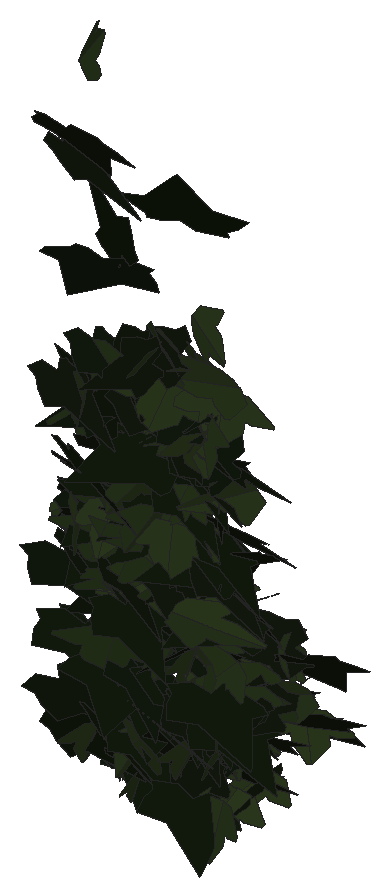
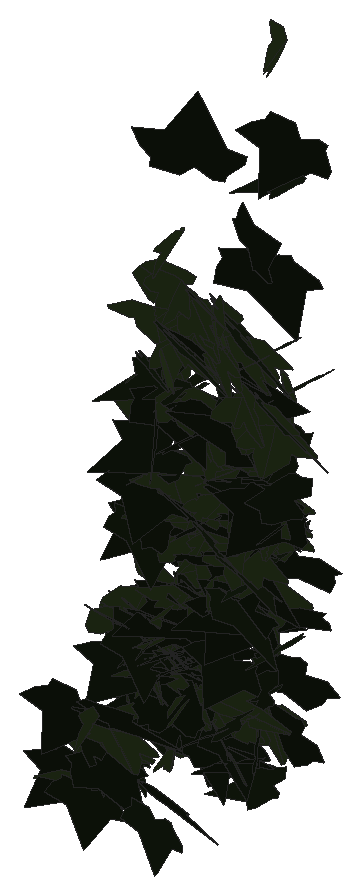
# SketchUp Ruby script. Lengths in millimetres.
U = 1.mm
M = Sketchup.active_model
def pt(a) = Geom::Point3d.new(a.map { |v| v * U })
def face(e, loops, mat)
  f = e.add_face(loops[0].map { |a| pt(a) })
  loops[1..].each { |l| e.add_face(l.map { |a| pt(a) }).erase! }
  f.material = f.back_material = mat if mat
  f
end
# faces: each face lists its corners as indices into pts; further lists are holes
def faces(e, pts, list, mat = nil) = list.each { |f| face(e, (f[0].is_a?(Array) ? f : [f]).map { |l| l.map { |i| pts[i] } }, mat) }
# xy, xz, yz: faces in a plane at the given z, y or x. An outline is a flat list of corners, or four numbers for a rectangle; further outlines are holes
def ring(l) = l.size == 4 ? [[l[0], l[1]], [l[2], l[1]], [l[2], l[3]], [l[0], l[3]]] : l.each_slice(2).to_a
def flat(e, list, mat, &to3) = list.each { |f| face(e, (f[0].is_a?(Array) ? f : [f]).map { |l| ring(l).map { |u, v| to3.(u, v) } }, mat) }
def xy(e, z, list, mat = nil) = flat(e, list, mat) { |x, y| [x, y, z] }
def xz(e, y, list, mat = nil) = flat(e, list, mat) { |x, z| [x, y, z] }
def yz(e, x, list, mat = nil) = flat(e, list, mat) { |y, z| [x, y, z] }
def lines(e, pts, list) = list.each { |a, b| e.add_line(pt(pts[a]), pt(pts[b])) }
# prism: a flat outline (further loops are holes) pulled along v
def prism(e, loops, v, mat = nil)
  f = face(e, loops, mat); d = Geom::Vector3d.new(v.map { |x| x * U })
  f.pushpull(f.normal.samedirection?(d) ? d.length : -d.length)
end
def box(e, o, s, mat = nil) = prism(e, [[o, [o[0] + s[0], o[1], o[2]], [o[0] + s[0], o[1] + s[1], o[2]], [o[0], o[1] + s[1], o[2]]]], [0, 0, s[2]], mat)
def at(x, y, z, deg = 0) = Geom::Transformation.translation(pt([x, y, z])) * Geom::Transformation.rotation(ORIGIN, Z_AXIS, deg.degrees)
def axes(o, x, y, z) = Geom::Transformation.new([*x, 0, *y, 0, *z, 0, *pt(o).to_a, 1])
def part(name) = M.definitions.add(name)
# library, detail: a bought-in or finely detailed component or shape, given as its bounding box
def library(name, o, s) = part(name).tap { |d| box(d.entities, o, s) }
def detail(e, o, s) = box(e.add_group.entities, o, s)
def put(e, d, t, mat = nil) = e.add_instance(d, t).tap { |i| i.material = mat if mat }
def group(e, t, mat = nil) = e.add_group.tap { |g| g.transformation = t; g.material = mat if mat }.entities
root = M.entities
M.materials.add("efeu1").color = [18, 25, 13]
M.materials.add("efeu2").color = [43, 57, 29]
c1 = part("ivyleaf_9")
p = [[39.1,54.8,31.7],[34.5,51.8,30.2],[-5.3,25.2,17.3],[-17.9,28.3,20.9],[-21.6,21.7,17],[-20.2,4.3,5.3],
  [-22.9,-0.3,2.5],[-17.1,-4,-0.6],[-2,-2.1,-1.2],[-0.7,-15.4,-10.1],[16.6,-22.3,-16.7],[21.1,-15.1,-12.5],
  [32.7,-10.7,-11],[46.1,-1.8,-6.6],[30.8,11.2,3.8]]
faces(c1.entities,p,[[0,1,2,3,4,5,6,7,8,9,10,11,12,13,14]],"efeu1")
c2 = part("ivyleaf_10")
p = [[0,12.8,-0.8],[-1.5,51.3,-10.9],[-4.9,51,-11.6],[-13.6,26.5,-7.3],[-13.2,15.9,-4.6],[-21.1,19.3,-7.2],
  [-29.5,16.3,-8.3],[-29.2,8.3,-6.2],[-19.7,-9.8,0.5],[-7.6,-13,4],[1,-12.2,5.8],[-0.4,51.1,-11.1],
  [-1.5,51.1,-10.9],[1,-12.4,5.9],[16.9,-12.4,3.5],[35.1,9.1,-5.1],[35,12.9,-6.1],[20.5,16.4,-4.9],
  [15.8,15,-3.8],[15.3,27.6,-7.1],[12.8,31.3,-7.8]]
faces(c2.entities,p,[[0,1,2,3,4,5,6,7,8,9,10],[11,12,0,13,14,15,16,17,18,19,20]],"efeu2")
put(root,c1,axes([3061,972.3,1635.7],[1.11104,-0.60833,-0.00442],[0.18227,0.09795,-0.83193],[1.14337,0.57552,0.13692]))
put(root,c1,axes([3073,929.3,1931.4],[0.51198,-0.71925,-0.46522],[-0.31436,0.43492,-0.7679],[1.59967,0.31566,-0.00201]))
put(root,c2,axes([3095.9,929.4,1935.7],[-1.34679,0.48513,0.2721],[-0.40759,0.16873,-0.8578],[-0.97701,-0.73914,-0.01723]))
put(root,c1,axes([3071.8,944.6,1785],[0.22855,-0.87259,0.06119],[0.01219,-0.06088,-0.88081],[1.66474,0.12024,-0.00195]))
put(root,c2,axes([3094.9,925.5,1684.9],[-0.36174,-0.88496,-0.00511],[0.00062,0.00516,-0.90514],[1.68428,-0.19007,-0.00076]))
put(root,c1,axes([3112.5,915.7,2059.2],[-1.31576,0.6085,-0.06336],[0.07292,-0.05235,-0.92089],[-1.16208,-0.69226,0.01395]))
put(root,c2,axes([3090.5,929.2,2034.6],[-1.18294,-0.64557,-0.1632],[0.34038,0.05319,-0.89158],[1.22074,-0.64042,0.09046]))
put(root,c1,axes([3058.2,928.1,1680.8],[0.22802,-0.13014,-0.86664],[1.59305,0.27606,0.07426],[0.49399,-0.83019,0.16055]))
put(root,c1,axes([3074.9,894.8,2090.1],[0.54567,-0.85198,-0.28202],[0.00984,0.29762,-0.89387],[1.70799,0.27047,0.09525]))
put(root,c2,axes([3088.3,929.8,1926.4],[1.70167,-0.0799,0.05219],[0.0972,-0.01482,-0.89762],[0.15343,0.89551,-0.01019]))
put(root,c1,axes([3084.1,933.4,1947.3],[1.61846,0.33248,-0.06095],[-0.10872,-0.02127,-0.91307],[-0.63407,0.8523,0.00099]))
put(root,c1,axes([3120.6,1097.6,1663.8],[-1.47036,0.30855,0.01572],[-0.04089,-0.01141,-0.8317],[-0.58657,-0.77265,0.01856]))
put(root,c2,axes([3102.9,891.1,2078.3],[0.7245,-0.79091,-0.40343],[-0.06508,0.42556,-0.86657],[1.68853,0.35576,0.1397]))
put(root,c2,axes([3100.7,886.1,1936.8],[0.35936,-0.41507,-0.79085],[0.11802,0.81247,-0.41162],[1.69576,0.03142,0.19624]))
put(root,c2,axes([3102.9,929.8,1928.9],[-1.33956,-0.59327,0.01785],[0.22886,-0.16965,-0.8969],[1.10619,-0.68333,0.20718]))
put(root,c1,axes([3093.5,884.1,2377.9],[1.73709,0.16773,-0.33496],[-0.65268,0.0191,-0.92489],[-0.28691,0.97206,0.07597]))
put(root,c1,axes([3079.3,905.2,1882],[-0.56523,-0.36346,-0.83752],[1.15093,0.5815,-0.46679],[1.30176,-0.67194,0.04905]))
put(root,c2,axes([3104.4,933.3,1801.8],[0.54825,0.78096,-0.33312],[-0.46526,-0.26058,-0.82231],[-1.54746,0.35503,0.12921]))
put(root,c1,axes([3110.6,1107.5,1633.5],[0.18597,0.77027,0.27647],[0.04997,0.27534,-0.7764],[-1.55675,0.10086,0.00811]))
put(root,c1,axes([3072.7,904,1738.3],[0.14565,-0.1347,-0.92948],[1.05057,0.76094,-0.06482],[1.44614,-0.53922,0.14071]))
put(root,c1,axes([3067.2,929.1,1966.6],[1.22331,-0.50011,0.43505],[0.86633,-0.10748,-0.79609],[0.91703,0.76867,0.17173]))
put(root,c1,axes([3082.7,906.4,1900.5],[1.00727,-0.69391,-0.2124],[-0.12161,0.2173,-0.86916],[1.37577,0.52725,0.07868]))
put(root,c1,axes([3086.3,963.9,1668.5],[0.14607,-0.13064,-0.83273],[1.33119,-0.45676,0.13612],[-0.89526,-0.7005,0.06654]))
put(root,c1,axes([3123.1,952,1829.2],[-0.2636,0.86615,-0.01475],[-0.29797,-0.03972,-0.86228],[-1.62155,-0.1335,0.16085]))
put(root,c1,axes([3117,908.7,2227.7],[0.90471,0.57918,-0.65463],[-0.8303,-0.48851,-0.749],[-1.4415,0.64489,0.02056]))
put(root,c1,axes([3080.1,899.8,2348.9],[1.09753,-0.76119,-0.19476],[0.03349,0.25404,-0.94077],[1.49499,0.55313,0.16406]))
put(root,c2,axes([3130.3,933.5,2066.3],[-0.60089,0.22129,0.83082],[-1.31041,0.465,-0.3855],[-0.98001,-0.75744,0.00606]))
put(root,c2,axes([3111.9,971.8,1651.5],[0.73007,-0.73576,0.02906],[0.02388,-0.02624,-0.82975],[1.40119,0.3838,-0.001]))
put(root,c1,axes([3138.8,901.2,2059.6],[-0.123,0.12449,0.9838],[-0.86939,0.87132,-0.14026],[-1.67514,-0.46135,0.00056]))
put(root,c1,axes([3120.6,959.4,1669.9],[0.19457,0.83622,-0.0593],[-0.01111,-0.05903,-0.84245],[-1.59546,0.10239,-0.00137]))
put(root,c1,axes([3098.2,905.3,1808.6],[-0.69692,-0.70373,-0.51272],[0.58025,0.41737,-0.79061],[1.55221,-0.47199,0.06534]))
put(root,c2,axes([3145,958.9,1708.5],[0.5784,0.03428,-0.94877],[-1.80391,0.06804,-0.30115],[0.10354,0.99393,0.05334]))
put(root,c1,axes([3133.9,923.6,1853.6],[0.04767,0.69432,0.56069],[-0.62264,0.52901,-0.64047],[-1.58025,-0.18749,0.26927]))
put(root,c1,axes([3098.5,928.2,1902],[0.13666,-0.89474,-0.00496],[-0.01012,0.00455,-0.8976],[1.70286,0.07183,-0.00494]))
put(root,c1,axes([3086.9,901.3,2000.8],[1.00367,-0.78971,0.23886],[0.19765,-0.21769,-0.94901],[1.55773,0.53644,-0.03348]))
put(root,c1,axes([3135.7,912.6,2244.2],[0.09116,-0.18226,1.01157],[-0.33332,0.99641,0.18782],[-1.92762,-0.18092,0.01536]))
put(root,c2,axes([3121.8,927.8,2054.8],[-1.52392,-0.43922,-0.06667],[0.10154,0.04135,-0.91321],[0.83938,-0.80242,-0.01057]))
put(root,c2,axes([3123.6,939.6,1880.2],[-1.65964,-0.15999,0.0083],[-0.00698,-0.02598,-0.88623],[0.30482,-0.87168,0.02489]))
put(root,c2,axes([3128.5,872.9,2477.3],[0.02596,-0.0121,1.00923],[-0.79646,0.9184,0.01667],[-1.748,-0.41864,0.00739]))
put(root,c1,axes([3110.7,953.2,1818.5],[1.31686,0.53596,0.01849],[0.00591,0.02618,-0.87502],[-1.02064,0.69167,0.01879]))
put(root,c2,axes([3129.7,895.4,1934.1],[-1.50138,-0.39575,0.18638],[-0.24418,-0.15811,-0.87876],[0.79592,-0.79502,0.08199]))
put(root,c1,axes([3111.1,907.3,1939.5],[1.41938,0.6399,0.01935],[0.02818,0.01246,-0.98269],[-1.21809,0.74594,-0.00019]))
put(root,c2,axes([3137,911.3,2119.3],[-1.607,0.10526,0.34407],[-0.67932,-0.13427,-0.83486],[-0.08643,-0.90184,0.16446]))
put(root,c1,axes([3097.2,935.3,1721.3],[1.12373,-0.62037,0.05149],[0.06616,-0.03799,-0.85643],[1.18289,0.59146,-0.00101]))
put(root,c1,axes([3132.4,918.3,1914.4],[-1.46169,-0.46735,0.06719],[-0.10838,-0.03568,-0.89903],[0.89204,-0.77013,0.00088]))
put(root,c1,axes([3110.7,976.4,1645.8],[-0.21903,-0.77726,-0.26],[0.12631,0.25285,-0.78526],[1.55472,-0.13004,0.02717]))
put(root,c1,axes([3103.7,914.4,2127.5],[0.51371,-0.87248,-0.2569],[-0.03673,0.26242,-0.9115],[1.73059,0.26455,0.05691]))
put(root,c1,axes([3138.6,919.1,1954.7],[-1.51094,-0.41525,0.13081],[-0.1992,-0.08203,-0.89562],[0.80429,-0.80041,0.02392]))
put(root,c2,axes([3117.8,958.1,1682.4],[1.32683,0.4648,0.13844],[0.06979,0.19121,-0.82664],[-0.92037,0.68457,0.1369]))
put(root,c2,axes([3132.1,923,1812.9],[-0.05377,-0.92668,0.01137],[0.00048,-0.01139,-0.92711],[1.76378,-0.02825,0.0006]))
put(root,c1,axes([3151.5,912.4,2131.1],[-1.07847,0.72273,0.07352],[-0.06021,0.06861,-0.91823],[-1.38129,-0.56728,-0.01738]))
put(root,c1,axes([3106.1,948.3,1824.4],[1.48155,0.22839,0.34224],[0.5744,0.18081,-0.80715],[-0.53221,0.83092,0.08157]))
put(root,c2,axes([3144.9,908.3,1951.1],[-1.56219,-0.25882,0.28159],[-0.52538,-0.06056,-0.86033],[0.50383,-0.86566,-0.024]))
put(root,c1,axes([3154,929.2,1857.8],[0.35816,0.19068,-0.91303],[-1.15512,-0.68222,-0.26758],[-1.34793,0.6353,-0.0133]))
put(root,c1,axes([3129.7,950.7,1755.1],[0.74558,0.7292,0.29822],[0.22493,0.27489,-0.82741],[-1.48242,0.40846,0.02444]))
put(root,c2,axes([3130.1,905.8,1949.7],[0.97186,0.72235,-0.26572],[-0.29912,-0.2143,-0.88461],[-1.43398,0.53427,0.00443]))
put(root,c2,axes([3123.6,929.1,1802.8],[0.12648,-0.47004,-0.76344],[0.16192,-0.75877,0.47458],[-1.69859,-0.10733,-0.01161]))
put(root,c2,axes([3144,892.5,1813.9],[-1.61379,-0.54917,0.14085],[-0.21586,-0.08397,-1.0102],[1.05719,-0.85544,0.00874]))
put(root,c1,axes([3111.5,964.5,1696.6],[0.82638,-0.73922,0.02209],[0.086,0.00095,-0.85641],[1.40489,0.43477,0.03943]))
put(root,c1,axes([3111.7,915.8,1704.7],[0.81271,-0.75705,0.14353],[0.16581,-0.11561,-0.86897],[1.45708,0.43541,0.01883]))
put(root,c1,axes([3132.8,967.3,1654.2],[-1.21543,-0.48621,-0.27967],[0.57464,0.05916,-0.79233],[0.89966,-0.69466,0.12827]))
put(root,c2,axes([3135.7,967.1,1675.2],[0.73068,-0.73868,0.14378],[0.16213,-0.11771,-0.83223],[1.42303,0.3927,0.02099]))
put(root,c1,axes([3117.1,944.3,1852.5],[0.64897,-0.82183,-0.03042],[0.09772,0.05414,-0.88715],[1.56212,0.33803,0.06813]))
put(root,c1,axes([3155.2,897.7,2031.3],[-0.07601,0.92139,0.12156],[0.03019,0.12233,-0.92202],[-1.76852,-0.03751,-0.02097]))
put(root,c2,axes([3151.2,931.1,1898.5],[1.5485,-0.00082,-0.37135],[-0.66747,0.29233,-0.76905],[0.23235,0.84524,0.26562]))
put(root,c1,axes([3153.8,962.4,1654.5],[0.07686,0.83589,-0.07013],[0.02354,-0.0708,-0.83671],[-1.59627,0.0392,-0.01572]))
put(root,c2,axes([3147.1,928.3,1652],[0.21499,-0.82793,-0.16248],[0.04035,0.16666,-0.8345],[1.60526,0.10669,0.04274]))
put(root,c1,axes([3157.4,936.6,1897.5],[-1.66892,-0.14765,-0.1341],[0.24926,0.02979,-0.88921],[0.2863,-0.8866,-0.00754]))
put(root,c2,axes([3139.7,899.1,1886.2],[-1.09838,-0.58599,-0.40281],[0.62694,0.23944,-0.82029],[1.19937,-0.66182,0.05989]))
put(root,c1,axes([3144.8,903.3,1775.8],[-0.97084,-0.73714,-0.09526],[0.07333,0.08916,-0.89623],[1.41269,-0.51121,-0.01895]))
put(root,c1,axes([3134.7,972.8,1673.8],[-0.11032,-0.84044,-0.02442],[0.02876,0.02343,-0.84233],[1.59994,-0.05837,0.01346]))
put(root,c2,axes([3151.1,941.6,1833],[-0.35364,-0.86964,0.05641],[0.04459,-0.06264,-0.88855],[1.65798,-0.18381,0.03593]))
put(root,c2,axes([3168.5,900.7,1705.4],[-1.21905,0.30898,0.61131],[-1.0852,0.22322,-0.71027],[-0.72232,-0.85682,0.03541]))
put(root,c1,axes([3114.8,916.2,2008.2],[0.69178,-0.13118,0.84205],[1.62042,0.09526,-0.35269],[-0.06974,0.91219,0.15792]))
put(root,c2,axes([3167.2,967.6,1694.2],[-0.11911,0.06884,-0.8475],[-0.65793,0.77433,0.08843],[1.4785,0.35012,-0.02893]))
put(root,c2,axes([3188,971.6,1665.5],[-0.73938,-0.14463,0.9129],[-1.64359,-0.29611,-0.41442],[0.62691,-0.9469,-0.00984]))
put(root,c2,axes([3164.9,909.8,1998.4],[-0.63705,-0.75707,0.42071],[-0.25793,-0.39969,-0.82709],[1.62808,-0.35956,0.03358]))
put(root,c2,axes([3158.1,917.5,1699.9],[-0.34064,-0.74572,0.42865],[0.08247,-0.4451,-0.75623],[1.63494,-0.13292,0.12746]))
put(root,c1,axes([3135.9,910.2,1886.6],[0.55716,-0.84359,0.13417],[0.09202,-0.12524,-0.89293],[1.62309,0.29668,0.00457]))
put(root,c2,axes([3161.6,965.8,1697.1],[-1.155,-0.60003,0.03088],[0.17435,-0.13579,-0.83812],[1.13012,-0.59229,0.16086]))
put(root,c1,axes([3180.9,930.2,1886.5],[-1.13105,0.6691,-0.0104],[0.01563,-0.00662,-0.89492],[-1.2735,-0.59434,-0.00174]))
put(root,c1,axes([3182.9,904.1,2032.6],[-1.60931,-0.26579,0.29779],[-0.48444,-0.17829,-0.8819],[0.58515,-0.87858,0.08887]))
put(root,c1,axes([3149.5,943,1827.7],[0.79769,-0.66792,-0.41325],[-0.38913,0.35948,-0.78838],[1.44329,0.46607,0.01585]))
put(root,c2,axes([3164.5,1104.8,1717],[1.59631,0.05762,-0.139],[-0.26508,-0.00058,-0.84068],[-0.10837,0.85019,0.00885]))
put(root,c1,axes([3187.6,893.7,2141.4],[-1.4242,0.55681,-0.11188],[0.13304,-0.09335,-0.93217],[-1.07269,-0.75085,0.03293]))
put(root,c1,axes([3173.8,944.5,1864.3],[-1.23353,-0.60345,0.08908],[-0.12575,-0.05977,-0.88557],[1.1541,-0.65149,-0.00127]))
put(root,c1,axes([3135.9,975.7,1665.4],[1.21496,-0.11524,0.5274],[1.02742,0.13923,-0.62301],[-0.00372,0.81626,0.18073]))
put(root,c1,axes([3185.4,1102.9,1677.3],[0.07121,0.71147,-0.43043],[-0.41802,-0.4071,-0.69201],[-1.52638,0.14468,0.16944]))
put(root,c2,axes([3195.2,923.6,1860.5],[-0.18017,0.25205,0.89208],[-1.16666,-0.6897,0.12982],[1.32347,-0.57366,0.23588]))
put(root,c2,axes([3164.5,925.2,2106.7],[-1.36271,0.46987,-0.34019],[0.25953,-0.38894,-0.8242],[-1.0731,-0.69075,0.23268]))
put(root,c1,axes([3193.6,958.3,1712.8],[-1.56715,-0.04598,0.22969],[-0.4293,-0.07081,-0.82281],[0.12026,-0.85193,0.05599]))
put(root,c1,axes([3156.9,916.4,1710.3],[0.07612,-0.83472,-0.27833],[-0.0461,0.27746,-0.83561],[1.67399,0.0456,-0.01036]))
put(root,c1,axes([3149.4,929.3,1972],[0.70584,-0.72019,-0.42667],[0.0183,0.4703,-0.78548],[1.59305,0.31369,0.19807]))
put(root,c1,axes([3156.3,918,1774],[0.01211,-0.90084,0.18203],[0.01621,-0.18197,-0.90083],[1.74905,0.00792,0.00709]))
put(root,c1,axes([3200.5,1101.8,1735.4],[-1.39841,0.04713,0.43865],[-0.83471,0.01411,-0.73618],[-0.09079,-0.85563,0.01202]))
put(root,c1,axes([3168,938,1746.2],[-0.89792,-0.85626,-0.04424],[0.05664,0.03411,-0.97759],[1.63083,-0.47263,0.0096]))
put(root,c1,axes([3159.2,894.8,1855.7],[-0.02229,-0.81416,-0.42223],[0.03045,0.42202,-0.8142],[1.74523,-0.01776,0.00881]))
put(root,c1,axes([3166.7,926.6,1668.1],[1.46044,0.18996,0.45125],[-0.83691,-0.10147,0.7905],[0.40971,-0.8844,0.00622]))
put(root,c2,axes([3177.8,911.5,2142.5],[0.17365,-0.94807,-0.05139],[0.00588,0.05192,-0.95242],[1.80701,0.09094,0.00804]))
put(root,c2,axes([3181.4,903.2,1966],[-0.53633,-0.82946,0.30019],[-0.08671,-0.30103,-0.87455],[1.67659,-0.28091,0.0508]))
put(root,c2,axes([3177.6,926.8,2110.1],[1.32292,-0.57535,-0.20468],[-0.20628,0.18896,-0.89924],[1.14378,0.69954,0.07456]))
put(root,c2,axes([3168.9,967.9,1690],[1.58126,-0.10721,0.01454],[0.06875,0.16876,-0.81989],[0.19409,0.81365,0.17197]))
put(root,c2,axes([3179.9,933.6,1800.4],[-0.48546,-0.85325,0.20204],[0.05036,-0.21781,-0.88644],[1.66804,-0.24175,0.08557]))
put(root,c1,axes([3158.3,907.4,2090.5],[0.74545,-0.71642,-0.47501],[-0.08606,0.50411,-0.79759],[1.63371,0.35345,0.17473]))
put(root,c1,axes([3155.4,958.7,1678.8],[1.27079,-0.50134,0.05059],[0.07282,-0.0333,-0.83497],[0.95624,0.6688,-0.00365]))
put(root,c1,axes([3203.9,945.4,1812.2],[-1.6489,0.11673,0.05794],[-0.11746,-0.02448,-0.87361],[-0.21844,-0.86797,0.03243]))
put(root,c2,axes([3180.6,971.7,1693.3],[-0.27205,0.81426,-0.16283],[0.00142,-0.1651,-0.82626],[-1.58038,-0.14032,0.02729]))
put(root,c1,axes([3195.9,920.4,1802.9],[0.11599,0.86553,0.07416],[0.05535,0.07227,-0.86735],[-1.65239,0.06318,-0.02385]))
put(root,c2,axes([3186.8,951.5,1663.8],[1.17588,-0.591,-0.00668],[-0.00464,0.00712,-0.85499],[1.12486,0.61784,0.00346]))
put(root,c2,axes([3211.6,914.6,2138.5],[-0.96662,0.2847,0.735],[-1.26727,0.31293,-0.58133],[-0.80277,-0.83681,0.03267]))
put(root,c2,axes([3177.8,919.8,1870.2],[-0.49445,-0.57015,-0.64392],[0.77713,0.51024,-0.61654],[1.44062,-0.47093,0.11158]))
put(root,c1,axes([3188.5,963.9,1685.9],[-0.86736,-0.69815,0.11065],[-0.082,-0.10397,-0.83348],[1.3428,-0.45731,0.02057]))
put(root,c1,axes([3184.2,962.6,1718.2],[-0.83458,-0.7312,-0.11466],[0.14403,0.08828,-0.8524],[1.40125,-0.44458,0.01932]))
put(root,c1,axes([3211.4,909.8,2153.7],[-1.47898,0.50984,-0.07614],[0.07205,-0.08091,-0.92824],[-0.97843,-0.77662,0.04673]))
put(root,c2,axes([3196.9,938.5,1867.8],[-1.23127,-0.6021,0.11233],[-0.04318,-0.13972,-0.87957],[1.16488,-0.64159,0.08613]))
put(root,c1,axes([3180.9,988.7,1681.7],[1.58527,-0.54876,0.10469],[-0.12707,0.08883,0.99677],[-1.05561,-0.83479,0.03724]))
put(root,c1,axes([3193.9,1112.4,1642.3],[0.60709,0.76835,0.04389],[-0.0304,0.05411,-0.83118],[-1.4644,0.31741,0.03545]))
put(root,c2,axes([3181,907.5,1908.6],[-0.9078,-0.58391,-0.49781],[0.77153,0.3059,-0.74724],[1.23989,-0.61786,0.10049]))
put(root,c1,axes([3203.4,951.8,1715.4],[-1.49501,-0.34598,0.03958],[-0.07238,-0.01185,-0.85833],[0.6588,-0.78643,-0.00448]))
put(root,c1,axes([3177.3,928,2035.6],[-0.64738,-0.58215,-0.63417],[0.55652,0.5632,-0.67384],[1.54096,-0.44797,-0.02306]))
put(root,c2,axes([3216.5,1086.5,1692.9],[0.43511,0.28388,-0.78081],[-1.50129,-0.18003,-0.29642],[-0.49633,0.79342,0.21211]))
put(root,c2,axes([3209.9,927.6,1745.3],[-1.46608,0.16838,0.33576],[-0.64277,0.02478,-0.78728],[-0.31286,-0.83995,0.04408]))
put(root,c2,axes([3168.7,927.5,2136.2],[-0.19122,0.01502,1.02934],[1.57536,-0.61371,0.08975],[1.16485,0.83246,0.0476]))
put(root,c2,axes([3192.2,975.3,1637.4],[-0.07416,0.78274,-0.29062],[-0.05137,-0.29196,-0.78274],[-1.58824,-0.02711,0.03889]))
put(root,c1,axes([3183,955.4,1742.6],[0.01035,-0.85844,0.11648],[0.04115,-0.11631,-0.85821],[1.64824,0.0083,0.0207]))
put(root,c2,axes([3199.1,1099,1729.4],[-0.19866,0.60674,0.59736],[-0.28659,0.57919,-0.61459],[-1.59494,-0.17965,0.03603]))
put(root,c1,axes([3212.2,1083.2,1695.3],[-0.65451,0.6801,-0.39933],[0.27216,-0.37465,-0.76122],[-1.47612,-0.37063,0.03672]))
put(root,c2,axes([3202.1,944.6,1711.5],[0.94317,-0.67511,-0.30872],[-0.09383,0.34044,-0.82362],[1.40972,0.47434,0.15173]))
put(root,c1,axes([3190.9,963,1731.2],[-0.30787,-0.83823,0.10063],[-0.00413,-0.10205,-0.85352],[1.60677,-0.16087,0.01709]))
put(root,c2,axes([3199.1,904.6,2109.9],[1.72619,0.16,-0.15561],[-0.29039,-0.03079,-0.92099],[-0.31002,0.91973,-0.00376]))
put(root,c1,axes([3226.5,922.2,2101.9],[-1.42825,0.53768,0.05749],[-0.18257,-0.0356,-0.91929],[-1.01282,-0.7518,0.08464]))
put(root,c1,axes([3236.1,903.5,2088.7],[-0.96843,0.50559,0.58216],[-0.98237,0.29481,-0.70719],[-1.09017,-0.71479,0.12011]))
put(root,c1,axes([3231.6,929.3,1905.5],[-1.36943,0.52157,0.2293],[-0.34226,0.14259,-0.88864],[-1.02891,-0.74161,-0.00959]))
put(root,c2,axes([3215,931.8,2037.7],[-0.97018,-0.71089,0.27947],[-0.14381,-0.28741,-0.86892],[1.44664,-0.50533,0.10105]))
put(root,c2,axes([3222.7,959.6,1711.9],[0.96007,-0.38406,-0.67799],[-0.81841,0.53634,-0.62376],[1.23674,0.65306,0.11355]))
put(root,c1,axes([3190.5,921.6,1889.8],[0.68888,-0.58741,-0.57975],[-0.23454,0.58749,-0.67219],[1.55314,0.34926,0.15563]))
put(root,c1,axes([3197.8,965.6,1722.7],[-0.56961,-0.69263,-0.40311],[0.30443,0.37002,-0.75453],[1.49452,-0.33935,0.00005]))
put(root,c1,axes([3180.3,910.4,1728],[0.34835,-0.59002,0.61117],[0.82274,-0.4735,-0.58658],[1.39178,0.42758,0.19378]))
put(root,c1,axes([3226.6,941.7,1730.4],[-1.46634,0.36327,-0.14568],[0.26249,-0.04903,-0.85169],[-0.69712,-0.78258,-0.01426]))
put(root,c1,axes([3185.1,947.9,1794.7],[1.60869,0.24851,0.29573],[0.54124,0.08117,-0.88103],[-0.49754,0.89181,-0.00222]))
put(root,c2,axes([3196.8,947,1806],[1.24285,0.48624,0.35895],[0.29598,0.37548,-0.79155],[-1.11153,0.64367,0.19059]))
put(root,c2,axes([3214.8,924.6,1706.8],[-0.16953,-0.87599,0.02683],[0.00041,-0.02699,-0.88051],[1.66797,-0.08903,0.00294]))
put(root,c2,axes([3204.2,906.2,1949.9],[1.71523,0.14198,0.03758],[0.07072,0.00565,-0.91235],[-0.27042,0.902,-0.0002]))
put(root,c1,axes([3238.4,917.8,2102.4],[-1.09076,0.7143,0.15475],[-0.21637,0.10713,-0.91555],[-1.37406,-0.5839,0.02133]))
put(root,c2,axes([3225.9,930.4,1799.5],[0.84057,-0.37291,-0.65544],[-0.62117,0.59023,-0.55574],[1.29382,0.52565,0.15902]))
put(root,c2,axes([3214.4,914,2000.7],[1.47331,-0.46189,-0.12351],[-0.14835,0.10997,-0.89983],[0.89778,0.77616,0.054]))
put(root,c1,axes([3218.3,932.1,1685.2],[-1.51749,-0.09498,-0.35517],[0.66883,0.0523,-0.80291],[0.20556,-0.87129,-0.00948]))
put(root,c2,axes([3216.6,923.7,1810.5],[0.01283,-0.87329,-0.03008],[0.10659,0.03045,-0.87151],[1.65962,0.0048,0.05621]))
put(root,c2,axes([3212.8,949.9,1752.1],[0.47656,0.79694,0.21061],[-0.20405,0.24973,-0.81751],[-1.55548,0.21141,0.17176]))
put(root,c2,axes([3211.7,932.4,1782],[0.10217,0.07302,-0.95829],[0.47839,0.92531,0.08459],[1.76545,-0.25496,0.03254]))
put(root,c1,axes([3205.8,948.4,1752.2],[0.15683,-0.6793,-0.52361],[-0.16762,0.51654,-0.68398],[1.62371,0.11894,-0.02004]))
put(root,c1,axes([3202.5,925.2,1994.5],[0.26019,-0.88224,-0.24414],[-0.04412,0.24343,-0.89266],[1.74163,0.13797,0.01386]))
put(root,c2,axes([3211,1112,1652.7],[1.22609,0.53007,0.03919],[0.06219,0.02196,-0.83426],[-1.00966,0.64504,-0.0038]))
put(root,c1,axes([3240.7,952.7,1691.7],[-1.19609,0.56719,-0.00148],[0.01502,0.00654,-0.8465],[-1.07937,-0.62843,-0.01014]))
put(root,c1,axes([3231.9,927,2029.9],[0.4174,0.72452,-0.53264],[-0.29799,-0.50911,-0.75699],[-1.6853,0.26946,0.00193]))
put(root,c1,axes([3207.6,962.4,1741.7],[-0.00842,-0.85306,-0.12076],[-0.01826,0.1208,-0.85301],[1.63962,-0.00303,-0.01012]))
put(root,c1,axes([3205.7,936.1,1737],[0.19139,-0.88852,-0.10206],[-0.04972,0.09974,-0.89407],[1.70143,0.10286,-0.01465]))
put(root,c2,axes([3217.4,938.3,1940.5],[1.46356,0.44717,-0.1306],[-0.18376,-0.0936,-0.88898],[-0.86735,0.77437,-0.03204]))
put(root,c2,axes([3227.8,964.6,1672.9],[0.16555,-0.66053,0.52545],[0.06312,-0.52515,-0.66565],[1.60514,0.08877,-0.02802]))
put(root,c1,axes([3220.3,902.5,2314.5],[1.71528,0.01452,0.45871],[-0.87345,0.03227,0.90069],[-0.00325,-1.01077,0.03534]))
put(root,c1,axes([3216.9,959.4,1758.8],[-0.26601,-0.85048,0.09091],[-0.0013,-0.09201,-0.86177],[1.62786,-0.13905,0.01417]))
put(root,c1,axes([3248.4,930.4,1922.2],[-1.16618,-0.38127,0.52399],[-0.87156,-0.25546,-0.7214],[0.87261,-0.7647,-0.02026]))
put(root,c1,axes([3215.5,1104.2,1655.8],[1.2874,0.44561,0.20761],[0.30579,0.13335,-0.80972],[-0.88423,0.6949,0.02225]))
put(root,c1,axes([3225.3,962.8,1732.4],[-0.66748,-0.75138,0.22692],[0.00094,-0.24876,-0.82291],[1.49382,-0.33558,0.10191]))
put(root,c1,axes([3247.8,992,1636.4],[-0.23497,0.75644,0.33418],[-0.14788,0.32578,-0.76612],[-1.56692,-0.14418,0.02219]))
put(root,c1,axes([3224.8,1095.2,1731],[1.25225,0.53032,-0.0035],[-0.00065,-0.00516,-0.84508],[-1.00932,0.65796,-0.0038]))
put(root,c1,axes([3239.8,967.5,1746.7],[0.38894,0.81878,0.07955],[-0.02792,0.08558,-0.84318],[-1.5654,0.20191,0.0348]))
put(root,c2,axes([3233,960,1700.4],[0.74018,-0.73348,-0.18883],[0.06388,0.22875,-0.81942],[1.44007,0.36686,0.13341]))
put(root,c1,axes([3218.6,926.9,2034.7],[0.33201,-0.91011,-0.0057],[-0.00777,0.00502,-0.92668],[1.73215,0.17447,-0.00307]))
put(root,c2,axes([3240.5,922.5,2073.1],[0.23728,-0.92554,-0.0414],[0.00351,0.04202,-0.93387],[1.76324,0.12446,0.00743]))
put(root,c2,axes([3235,952.9,1731.7],[1.35376,-0.45927,0.00572],[0.01184,-0.00091,-0.84669],[0.87408,0.71133,0.00261]))
put(root,c1,axes([3217.9,921,2044.8],[0.65668,-0.85898,-0.14585],[-0.02628,0.15146,-0.92468],[1.658,0.34261,0.04311]))
put(root,c1,axes([3212.6,954.4,1671.7],[1.43604,0.12845,0.38636],[0.68365,0.17302,-0.75904],[-0.36481,0.82986,0.09845]))
put(root,c2,axes([3216.3,962.7,1712.2],[-0.63166,-0.22153,-0.74813],[1.35145,0.25115,-0.38939],[0.61536,-0.77896,0.08722]))
put(root,c1,axes([3260.6,959.5,1772.5],[-1.58467,-0.13282,0.17577],[-0.27772,-0.18234,-0.82902],[0.31414,-0.83122,0.15377]))
put(root,c1,axes([3253.3,924.9,2001],[0.26424,-0.01392,-1.00697],[-1.53131,0.60978,-0.11937],[1.15266,0.81329,0.07226]))
put(root,c1,axes([3235,903.7,1659.3],[-0.67703,-0.80751,-0.25845],[0.16004,0.24529,-0.88214],[1.60568,-0.36493,-0.02105]))
put(root,c2,axes([3237.9,961.9,1714.2],[-1.09647,0.44534,-0.42847],[0.19254,-0.50991,-0.66602],[-1.16029,-0.50546,0.29438]))
put(root,c2,axes([3242.4,965.9,1712.9],[-0.99611,0.66157,0.02309],[-0.05113,0.00818,-0.84342],[-1.25882,-0.52383,0.01599]))
put(root,c1,axes([3257,941.8,1772.6],[-0.02155,0.85999,-0.10711],[-0.13275,-0.10767,-0.85717],[-1.64404,-0.00258,0.07062]))
put(root,c2,axes([3243.9,909.9,2155.3],[-1.37346,0.5894,0.02654],[-0.04742,0.01145,-0.93174],[-1.12188,-0.72205,0.00689]))
put(root,c2,axes([3247,902.2,2073.7],[-0.68501,-0.83798,-0.1657],[0.25282,0.12272,-0.90912],[1.60594,-0.37675,0.07244]))
put(root,c1,axes([3256.8,940.4,1870.5],[0.33896,0.86314,0.16315],[-0.10833,0.17746,-0.8767],[-1.66829,0.16385,0.09008]))
put(root,c2,axes([3249.8,921,1715.3],[0.01898,-0.53866,-0.7302],[0.08709,0.72962,-0.5376],[1.72475,-0.03091,0.03518]))
put(root,c2,axes([3256.5,983.2,1659.8],[0.98035,0.41241,-0.51416],[-0.74208,-0.33546,-0.6597],[-1.01141,0.64588,-0.01434]))
put(root,c1,axes([3267.9,933.9,1868.2],[-1.60668,-0.25635,0.1619],[-0.29479,-0.04711,-0.88227],[0.49606,-0.85829,0.00007]))
put(root,c1,axes([3249.1,937.7,1924.1],[0.91198,0.76139,0.02592],[0.01654,0.02515,-0.89961],[-1.44982,0.47922,0.00604]))
put(root,c2,axes([3242.8,933.2,1894.1],[0.56131,0.83891,0.11528],[0.02803,0.11697,-0.8889],[-1.61137,0.29426,0.02469]))
put(root,c1,axes([3238,957,1749.8],[0.95679,-0.52836,-0.45355],[-0.52012,0.3648,-0.7279],[1.21892,0.5704,0.04541]))
put(root,c2,axes([3259.4,926.1,1810.7],[1.28774,-0.45975,-0.34866],[-0.52333,0.21546,-0.81774],[0.96542,0.73003,0.02178]))
put(root,c1,axes([3274.4,912.1,2051.7],[-1.30648,0.64382,-0.03567],[0.04221,-0.02849,-0.94112],[-1.22647,-0.6868,0.0056]))
put(root,c2,axes([3280.2,892.5,2150.3],[0.80424,-0.0171,-0.82934],[-1.46912,0.33266,-0.40018],[0.578,0.86931,0.13682]))
put(root,c1,axes([3276.1,950,1774],[-1.48624,0.37303,0.01141],[-0.02559,-0.00168,-0.86541],[-0.70983,-0.781,0.00731]))
put(root,c2,axes([3251,954.3,1790.4],[-1.31185,-0.48487,-0.23796],[0.46973,0.06042,-0.83802],[0.91435,-0.7267,0.0891]))
put(root,c2,axes([3258.3,936,1656.5],[0.80998,0.58591,-0.52228],[-0.56991,-0.42798,-0.72413],[-1.38084,0.52032,-0.0075]))
put(root,c2,axes([3238.8,905.9,2084.7],[1.43701,-0.33149,0.41588],[0.73334,-0.15679,-0.82455],[0.69764,0.84763,0.01012]))
put(root,c1,axes([3271.9,945.2,1655.7],[-0.67067,0.76153,-0.1147],[0.12576,-0.09578,-0.83888],[-1.46029,-0.358,-0.01957]))
put(root,c2,axes([3254.3,894.5,2206.7],[-0.28258,0.8548,0.34443],[-0.11169,0.3394,-0.8676],[-1.7504,-0.15965,-0.00024]))
put(root,c1,axes([3239.6,932.3,1913.5],[0.44578,-0.82469,-0.26147],[0.02553,0.27431,-0.85318],[1.64635,0.21905,0.08403]))
put(root,c1,axes([3292.5,960.7,1754.9],[-1.03841,0.49114,0.42681],[-0.88449,0.09571,-0.70423],[-0.86674,-0.68608,0.2073]))
put(root,c1,axes([3245.8,942.7,1884.5],[1.59485,-0.20634,-0.25437],[-0.4514,0.09964,-0.86216],[0.42993,0.87006,0.03841]))
put(root,c2,axes([3275.3,963.8,1762.8],[-1.43222,-0.30302,0.26361],[-0.41372,-0.16347,-0.80848],[0.64275,-0.78043,0.067]))
put(root,c1,axes([3239.4,918,2050.2],[1.60389,-0.32966,-0.17543],[-0.05622,0.37283,-0.84249],[0.70849,0.77587,0.3303]))
put(root,c2,axes([3234.3,902.4,1867.8],[-0.48961,-0.1989,-0.85564],[1.60679,0.19035,-0.29809],[0.46192,-0.87296,0.12996]))
put(root,c1,axes([3240.3,927.9,1967.5],[1.71074,-0.03814,0.0874],[0.17626,0.15182,-0.88625],[0.04322,0.89026,0.15488]))
put(root,c1,axes([3255.9,963.8,1713.7],[1.32542,0.46459,0.12241],[-0.00046,0.21591,-0.81806],[-0.91439,0.67333,0.17785]))
put(root,c2,axes([3285.6,919.7,2016.4],[0.32327,0.36987,-0.83067],[-1.29515,-0.50876,-0.36569],[-1.1478,0.67825,0.17868]))
put(root,c1,axes([3248.1,933.4,1945.4],[0.37162,-0.89312,-0.04346],[0.00493,0.04504,-0.91414],[1.7018,0.1949,0.01214]))
put(root,c1,axes([3254,911.8,1781.3],[-0.46833,-0.68822,-0.55777],[0.40536,0.51595,-0.73058],[1.63653,-0.32475,0.02134]))
put(root,c2,axes([3267.7,940.1,1776.3],[-1.26564,-0.522,-0.17987],[0.37167,0.041,-0.84098],[0.98287,-0.68768,0.0864]))
put(root,c2,axes([3264.1,912.9,2118.7],[1.71805,0.27085,-0.02157],[-0.03672,-0.01073,-0.94246],[-0.51581,0.90291,-0.00473]))
put(root,c1,axes([3252.8,934.9,1744],[-0.14752,-0.75806,-0.52624],[0.38847,0.50093,-0.75166],[1.7128,-0.17891,0.12516]))
put(root,c2,axes([3262.9,905.7,1656.2],[1.4199,-0.58457,0.23749],[0.35598,-0.14635,-0.9478],[1.14689,0.76915,0.00016]))
